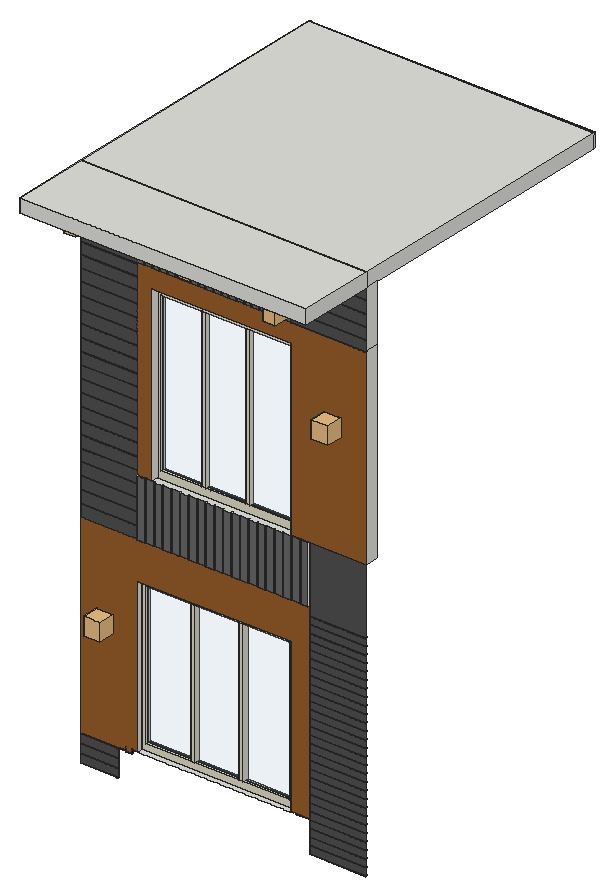
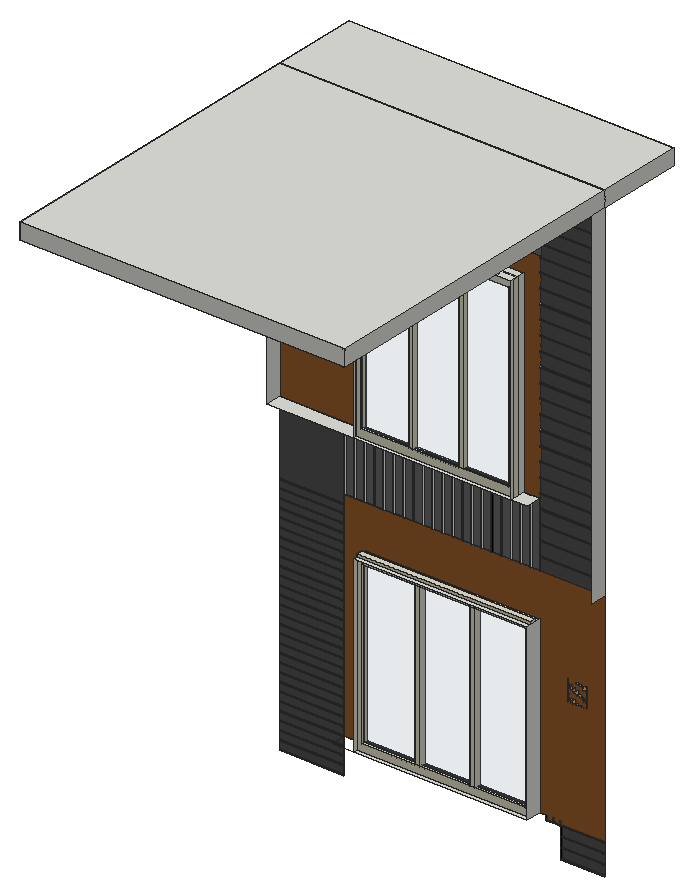
# SketchUp Ruby script. Lengths in inches.
U = 1.inch
M = Sketchup.active_model
def pt(a) = Geom::Point3d.new(a.map { |v| v * U })
def face(e, loops, mat)
  f = e.add_face(loops[0].map { |a| pt(a) })
  loops[1..].each { |l| e.add_face(l.map { |a| pt(a) }).erase! }
  f.material = f.back_material = mat if mat
  f
end
# faces: each face lists its corners as indices into pts; further lists are holes
def faces(e, pts, list, mat = nil) = list.each { |f| face(e, (f[0].is_a?(Array) ? f : [f]).map { |l| l.map { |i| pts[i] } }, mat) }
# xy, xz, yz: faces in a plane at the given z, y or x. An outline is a flat list of corners, or four numbers for a rectangle; further outlines are holes
def ring(l) = l.size == 4 ? [[l[0], l[1]], [l[2], l[1]], [l[2], l[3]], [l[0], l[3]]] : l.each_slice(2).to_a
def flat(e, list, mat, &to3) = list.each { |f| face(e, (f[0].is_a?(Array) ? f : [f]).map { |l| ring(l).map { |u, v| to3.(u, v) } }, mat) }
def xy(e, z, list, mat = nil) = flat(e, list, mat) { |x, y| [x, y, z] }
def xz(e, y, list, mat = nil) = flat(e, list, mat) { |x, z| [x, y, z] }
def yz(e, x, list, mat = nil) = flat(e, list, mat) { |y, z| [x, y, z] }
def lines(e, pts, list) = list.each { |a, b| e.add_line(pt(pts[a]), pt(pts[b])) }
# prism: a flat outline (further loops are holes) pulled along v
def prism(e, loops, v, mat = nil)
  f = face(e, loops, mat); d = Geom::Vector3d.new(v.map { |x| x * U })
  f.pushpull(f.normal.samedirection?(d) ? d.length : -d.length)
end
def box(e, o, s, mat = nil) = prism(e, [[o, [o[0] + s[0], o[1], o[2]], [o[0] + s[0], o[1] + s[1], o[2]], [o[0], o[1] + s[1], o[2]]]], [0, 0, s[2]], mat)
def at(x, y, z, deg = 0) = Geom::Transformation.translation(pt([x, y, z])) * Geom::Transformation.rotation(ORIGIN, Z_AXIS, deg.degrees)
def axes(o, x, y, z) = Geom::Transformation.new([*x, 0, *y, 0, *z, 0, *pt(o).to_a, 1])
def part(name) = M.definitions.add(name)
# library, detail: a bought-in or finely detailed component or shape, given as its bounding box
def library(name, o, s) = part(name).tap { |d| box(d.entities, o, s) }
def detail(e, o, s) = box(e.add_group.entities, o, s)
def put(e, d, t, mat = nil) = e.add_instance(d, t).tap { |i| i.material = mat if mat }
def group(e, t, mat = nil) = e.add_group.tap { |g| g.transformation = t; g.material = mat if mat }.entities
root = M.entities
M.materials.add("Glass").color = [171, 209, 242]
M.materials["Glass"].alpha = 0.09
M.materials.add("Plastic_SSS_01_White").color = [225, 221, 201]
M.materials.add("[0010_Snow]").color = [255, 250, 250]
M.materials.add("[0134_DimGray]").color = [105, 105, 105]
M.materials.add("[0135_DarkGray]").color = [81, 81, 81]
M.materials.add("[0137_Black]").color = [0, 0, 0]
M.materials.add("[Wood Floor Dark]1").color = [153, 94, 42]
c1 = part("Window frame")
xy(c1.entities,0,[[[104.47,83.98,176.47,131.98],[106.47,85.98,174.47,129.98]],[127.47,85.98,129.47,129.98],[150.47,85.98,152.47,129.98]],"Plastic_SSS_01_White")
xy(c1.entities,2,[[[104.47,83.98,176.47,131.98],[106.47,85.98,174.47,129.98]],[127.47,85.98,129.47,129.98],[150.47,85.98,152.47,129.98]],"Plastic_SSS_01_White")
xz(c1.entities,83.98,[[104.47,0,176.47,2]],"Plastic_SSS_01_White")
xz(c1.entities,85.98,[[106.47,0,127.47,2],[127.47,0,129.47,2],[129.47,0,150.47,2],[150.47,0,152.47,2],[152.47,0,174.47,2]],"Plastic_SSS_01_White")
xz(c1.entities,129.98,[[106.47,0,127.47,2],[127.47,0,129.47,2],[129.47,0,150.47,2],[150.47,0,152.47,2],[152.47,0,174.47,2]],"Plastic_SSS_01_White")
xz(c1.entities,131.98,[[104.47,0,176.47,2]],"Plastic_SSS_01_White")
yz(c1.entities,104.47,[[83.98,0,131.98,2]],"Plastic_SSS_01_White")
yz(c1.entities,106.47,[[85.98,0,129.98,2]],"Plastic_SSS_01_White")
yz(c1.entities,127.47,[[85.98,0,129.98,2]],"Plastic_SSS_01_White")
yz(c1.entities,129.47,[[85.98,0,129.98,2]],"Plastic_SSS_01_White")
yz(c1.entities,150.47,[[85.98,0,129.98,2]],"Plastic_SSS_01_White")
yz(c1.entities,152.47,[[85.98,0,129.98,2]],"Plastic_SSS_01_White")
yz(c1.entities,174.47,[[85.98,0,129.98,2]],"Plastic_SSS_01_White")
yz(c1.entities,176.47,[[83.98,0,131.98,2]],"Plastic_SSS_01_White")
c2 = part("Window pane")
box(c2.entities,[0,0,0],[67.88,44,0.5])
c3 = part("Glazed window assembly")
put(c3.entities,c1,at(-104.47,-83.98,0))
put(c3.entities,c2,at(2,2,0.7),"Glass")
c4 = part("window")
p = [[-596.28,88.12,20.39],[-668.28,88.12,20.39]]
lines(c4.entities,p,[[0,1]])
put(c4.entities,c3,axes([-668.28,88.12,20.39],[1,0,0],[0,0,1],[0,-1,0]))
c5 = library("Spot Light",[-5.1,-5.1,-11.05],[10.2,10.2,11.05])
c6 = library("Spot Light\#1",[-5.1,-5.1,-11.05],[10.2,10.2,11.05])
c7 = library("Sphere Light\#2",[-7.69,-7.69,-7.69],[15.38,15.38,15.38])
c8 = library("Sphere Light",[-0.01,-0.01,-0.01],[0.02,0.02,0.02])
c9 = library("Sphere Light\#1",[-0.01,-0.01,-0.01],[0.02,0.02,0.02])
xy(root,272.3,[[144.5,47.5,180,48]],"[0135_DarkGray]")
xy(root,272.8,[[144.5,47.5,180,48]],"[0135_DarkGray]")
xy(root,272.95,[[0,47.5,24,48]],"[0135_DarkGray]")
xy(root,273.45,[[0,47.5,24,48]],"[0135_DarkGray]")
xy(root,277.1,[[144.5,47.5,180,48]],"[0135_DarkGray]")
xy(root,277.6,[[144.5,47.5,180,48]],"[0135_DarkGray]")
xy(root,278.45,[[0,47.5,24,48]],"[0135_DarkGray]")
xy(root,278.95,[[0,47.5,24,48]],"[0135_DarkGray]")
xy(root,281.9,[[144.5,47.5,180,48]],"[0135_DarkGray]")
xy(root,282.4,[[144.5,47.5,180,48]],"[0135_DarkGray]")
xy(root,283.95,[[0,47.5,24,48]],"[0135_DarkGray]")
xy(root,284.45,[[0,47.5,24,48]],"[0135_DarkGray]")
xy(root,286.7,[[144.5,47.5,180,48]],"[0135_DarkGray]")
xy(root,287.2,[[144.5,47.5,180,48]],"[0135_DarkGray]")
xy(root,289.45,[[0,47.5,24,48]],"[0135_DarkGray]")
xy(root,291.5,[[144.5,47.5,180,48]],"[0135_DarkGray]")
xy(root,292,[[32.5,47.5,36,47.5,36,48,36.5,48,36.5,47.5,40,47.5,40,48,40.5,48,40.5,47.5,44,47.5,44,48,44.5,48,44.5,47.5,48,47.5,48,48,48.5,48,48.5,47.5,52,47.5,52,48,52.5,48,52.5,47.5,56,47.5,56,48,56.5,48,56.5,47.5,60,47.5,60,48,60.5,48,60.5,47.5,64,47.5,64,48,64.5,48,64.5,47.5,68,47.5,68,48,68.5,48,68.5,47.5,72,47.5,72,48,72.5,48,72.5,47.5,76,47.5,76,48,76.5,48,76.5,47.5,80,47.5,80,48,80.5,48,80.5,47.5,84,47.5,84,48,84.5,48,84.5,47.5,88,47.5,88,48,88.5,48,88.5,47.5,92,47.5,92,48,92.5,48,92.5,47.5,96,47.5,96,48,96.5,48,96.5,47.5,100,47.5,100,48,100.5,48,100.5,47.5,104,47.5,104,48,104.5,48,104.5,47.5,108,47.5,108,48,108.5,48,108.5,47.5,112,47.5,112,48,112.5,48,112.5,47.5,116,47.5,116,48,116.5,48,116.5,47.5,120,47.5,120,48,120.5,48,120.5,47.5,124,47.5,124,48,124.5,48,124.5,47.5,128,47.5,128,48,128.5,48,128.5,47.5,132,47.5,132,56.5,36,56.5,36,48,32.5,48],[132.5,47.5,136,48],[136.5,47.5,140,48],[140.5,47.5,144,48]])
xy(root,292,[[144.5,47.5,180,48]],"[0135_DarkGray]")
xy(root,296.3,[[144.5,47.5,180,48]],"[0135_DarkGray]")
xy(root,296.8,[[144.5,47.5,180,48]],"[0135_DarkGray]")
xy(root,301.1,[[144.5,47.5,180,48]],"[0135_DarkGray]")
xy(root,301.6,[[144.5,47.5,180,48]],"[0135_DarkGray]")
xy(root,305.9,[[144.5,47.5,180,48]],"[0135_DarkGray]")
xy(root,306.4,[[144.5,47.5,180,48]],"[0135_DarkGray]")
xy(root,310.7,[[144.5,47.5,180,48]],"[0135_DarkGray]")
xy(root,311.2,[[144.5,47.5,180,48]],"[0135_DarkGray]")
xy(root,315.5,[[144.5,47.5,180,48]],"[0135_DarkGray]")
xy(root,316,[[144.5,47.5,180,48]],"[0135_DarkGray]")
xy(root,320.3,[[144.5,47.5,180,48]],"[0135_DarkGray]")
xy(root,320.8,[[144.5,47.5,180,48]],"[0135_DarkGray]")
xy(root,325.1,[[144.5,47.5,180,48]],"[0135_DarkGray]")
xy(root,325.6,[[144.5,47.5,180,48]],"[0135_DarkGray]")
xy(root,329.9,[[144.5,47.5,180,48]],"[0135_DarkGray]")
xy(root,330.4,[[144.5,47.5,180,48]],"[0135_DarkGray]")
xy(root,334.7,[[144.5,47.5,180,48]],"[0135_DarkGray]")
xy(root,335.2,[[144.5,47.5,180,48]],"[0135_DarkGray]")
xy(root,339.5,[[144.5,47.5,180,48]],"[0135_DarkGray]")
xy(root,340,[[144.5,47.5,180,48]],"[0135_DarkGray]")
xy(root,344.3,[[144.5,47.5,180,48]],"[0135_DarkGray]")
xy(root,344.8,[[144.5,47.5,180,48]],"[0135_DarkGray]")
xy(root,349.1,[[144.5,47.5,180,48]],"[0135_DarkGray]")
xy(root,349.6,[[144.5,47.5,180,48]],"[0135_DarkGray]")
xy(root,353.9,[[144.5,47.5,180,48]],"[0135_DarkGray]")
xy(root,354.4,[[144.5,47.5,180,48]],"[0135_DarkGray]")
xy(root,358.7,[[144.5,47.5,180,48]],"[0135_DarkGray]")
xy(root,359.2,[[144.5,47.5,180,48]],"[0135_DarkGray]")
xy(root,363.5,[[144.5,47.5,180,48]],"[0135_DarkGray]")
xy(root,364,[[144.5,47.5,180,48]],"[0135_DarkGray]")
xy(root,368.3,[[144.5,47.5,180,48]],"[0135_DarkGray]")
xy(root,368.8,[[144.5,47.5,180,48]],"[0135_DarkGray]")
xy(root,373.1,[[144.5,47.5,180,48]],"[0135_DarkGray]")
xy(root,373.6,[[144.5,47.5,180,48]],"[0135_DarkGray]")
xy(root,377.9,[[144.5,47.5,180,48]],"[0135_DarkGray]")
xy(root,378.4,[[144.5,47.5,180,48]],"[0135_DarkGray]")
xy(root,382.7,[[144.5,47.5,180,48]],"[0135_DarkGray]")
xy(root,383.2,[[144.5,47.5,180,48]],"[0135_DarkGray]")
xy(root,387.5,[[144.5,47.5,180,48]],"[0135_DarkGray]")
xy(root,388,[[36,48,132,56.5]])
xy(root,388,[[144.5,47.5,180,48]],"[0135_DarkGray]")
xy(root,392.3,[[144.5,47.5,180,48]],"[0135_DarkGray]")
xy(root,392.8,[[144.5,47.5,180,48]],"[0135_DarkGray]")
xy(root,397.1,[[144.5,47.5,180,48]],"[0135_DarkGray]")
xy(root,397.6,[[144.5,47.5,180,48]],"[0135_DarkGray]")
xy(root,401.9,[[144.5,47.5,180,48]],"[0135_DarkGray]")
xy(root,402.4,[[144.5,47.5,180,48]],"[0135_DarkGray]")
xy(root,406.7,[[144.5,47.5,180,48]],"[0135_DarkGray]")
xy(root,407.2,[[144.5,47.5,180,48]],"[0135_DarkGray]")
xy(root,412,[[35.8125,47.5,40.73,48],[41.23,47.5,46.15,48],[46.65,47.5,51.57,48],[52.07,47.5,56.99,48],[57.49,47.5,62.41,48],
  [62.91,47.5,67.82,48],[68.32,47.5,73.24,48],[73.74,47.5,78.66,48],[79.16,47.5,84.08,48],[84.58,47.5,89.5,48],
  [90,47.5,94.92,48],[95.42,47.5,100.34,48],[100.84,47.5,105.76,48],[106.26,47.5,111.18,48],[111.68,47.5,116.59,48],
  [117.09,47.5,122.01,48],[122.51,47.5,127.43,48],[127.93,47.5,132.85,48],[133.35,47.5,138.27,48],[138.77,47.5,143.6875,48]],"[0010_Snow]")
xy(root,419.32,[[0,48,35.3125,48.5]],"[0010_Snow]")
xy(root,419.82,[[0,48,35.3125,48.5]],"[0010_Snow]")
xy(root,427.15,[[0,48,35.3125,48.5]],"[0010_Snow]")
xy(root,427.65,[[0,48,35.3125,48.5]],"[0010_Snow]")
xy(root,434.98,[[0,48,35.3125,48.5]],"[0010_Snow]")
xy(root,435.48,[[0,48,35.3125,48.5]],"[0010_Snow]")
xy(root,442.8,[[0,48,35.3125,48.5]],"[0010_Snow]")
xy(root,443.3,[[0,48,35.3125,48.5]],"[0010_Snow]")
xy(root,448,[[35.8125,47.5,40.73,48],[41.23,47.5,46.15,47.5,46.15,48,46.65,48,46.65,47.5,51.57,47.5,51.57,48,52.07,48,52.07,47.5,56.99,47.5,56.99,48,57.49,48,57.49,47.5,62.41,47.5,62.41,48,62.91,48,62.91,47.5,67.82,47.5,67.82,48,68.32,48,68.32,47.5,73.24,47.5,73.24,48,73.74,48,73.74,47.5,78.66,47.5,78.66,48,79.16,48,79.16,47.5,84.08,47.5,84.08,48,84.58,48,84.58,47.5,89.5,47.5,89.5,48,90,48,90,47.5,94.92,47.5,94.92,48,95.42,48,95.42,47.5,100.34,47.5,100.34,48,100.84,48,100.84,47.5,105.76,47.5,105.76,48,106.26,48,106.26,47.5,111.18,47.5,111.18,48,111.68,48,111.68,47.5,116.59,47.5,116.59,48,117.09,48,117.09,47.5,122.01,47.5,122.01,48,122.51,48,122.51,47.5,127.43,47.5,127.43,48,127.93,48,127.93,47.5,132.85,47.5,132.85,48,132,48,132,56.5,44.8,56.5,44.8,48,41.23,48],[133.35,47.5,138.27,48],[138.77,47.5,143.6875,48],[144.5,47.5,180,48],
  [35.8125,48,44.8,56.5],[132,48,180,56.5]])
xy(root,450.625,[[0,48,35.3125,48.5]],"[0010_Snow]")
xy(root,451.125,[[0,48,35.3125,48.5]],"[0010_Snow]")
xy(root,458.45,[[0,48,35.3125,48.5]],"[0010_Snow]")
xy(root,458.95,[[0,48,35.3125,48.5]],"[0010_Snow]")
xy(root,466.28,[[0,48,35.3125,48.5]],"[0010_Snow]")
xy(root,466.78,[[0,48,35.3125,48.5]],"[0010_Snow]")
xy(root,474.1,[[0,48,35.3125,48.5]],"[0010_Snow]")
xy(root,474.6,[[0,48,35.3125,48.5]],"[0010_Snow]")
xy(root,481.92,[[0,48,35.3125,48.5]],"[0010_Snow]")
xy(root,482.42,[[0,48,35.3125,48.5]],"[0010_Snow]")
xy(root,489.75,[[0,48,35.3125,48.5]],"[0010_Snow]")
xy(root,490.25,[[0,48,35.3125,48.5]],"[0010_Snow]")
xy(root,497.58,[[0,48,35.3125,48.5]],"[0010_Snow]")
xy(root,498.08,[[0,48,35.3125,48.5]],"[0010_Snow]")
xy(root,505.4,[[0,48,35.3125,48.5]],"[0010_Snow]")
xy(root,505.9,[[0,48,35.3125,48.5]],"[0010_Snow]")
xy(root,513.22,[[0,48,35.3125,48.5]],"[0010_Snow]")
xy(root,513.72,[[0,48,35.3125,48.5]],"[0010_Snow]")
xy(root,521.05,[[0,48,35.3125,48.5]],"[0010_Snow]")
xy(root,521.55,[[0,48,35.3125,48.5]],"[0010_Snow]")
xy(root,528.875,[[0,48,35.3125,48.25]],"[0010_Snow]")
xy(root,529.375,[[0,48,35.3125,48.25]],"[0010_Snow]")
xy(root,536.7,[[0,48,35.3125,48.25]],"[0010_Snow]")
xy(root,537.2,[[0,48,35.3125,48.25]],"[0010_Snow]")
xy(root,544.55,[[0,48,35.3125,48.5]],"[0010_Snow]")
xy(root,545.03,[[0,48,35.3125,48.5]],"[0010_Snow]")
xy(root,552.35,[[0,48,35.3125,48.5]],"[0010_Snow]")
xy(root,552.85,[[0,48,35.3125,48.5]],"[0010_Snow]")
xy(root,556.5,[[44.8,48,132,56.5]])
xy(root,560.17,[[0,48,35.3125,48.5]],"[0010_Snow]")
xy(root,560.67,[[0,48,35.3125,48.5]],"[0010_Snow]")
xy(root,567.5,[[0,48,35.3125,48.5]],"[0010_Snow]")
xy(root,568,[[0,48,35.3125,48.5],[132,48,180,48.5]],"[0010_Snow]")
xy(root,568.5,[[39.65,48,40.15,48.5],[44.48,48,44.98,48.5],[49.32,48,49.82,48.5],[54.15,48,54.65,48.5],[58.98,48,59.48,48.5],
  [63.82,48,64.32,48.5],[68.65,48,69.15,48.5],[73.49,48,73.99,48.5],[78.32,48,78.82,48.5],[83.16,48,83.66,48.5],
  [87.99,48,88.49,48.5],[92.83,48,93.33,48.5],[97.66,48,98.16,48.5],[102.49,48,102.99,48.5],[107.33,48,107.83,48.5],
  [112.16,48,112.66,48.5],[117,48,117.5,48.5],[121.83,48,122.33,48.5],[126.67,48,127.17,48.5],[132,48,180,48.5]],"[0010_Snow]")
xy(root,574.5,[[0,48,35.3125,48.5],[132,48,180,48.5]],"[0010_Snow]")
xy(root,575,[[0,48,35.3125,48.5],[132,48,180,48.5]],"[0010_Snow]")
xy(root,582,[[0,48,35.3125,48.5],[132,48,180,48.5]],"[0010_Snow]")
xy(root,582.5,[[0,48,35.3125,48.5],[132,48,180,48.5]],"[0010_Snow]")
xy(root,589.5,[[0,48,35.3125,48.5],[132,48,180,48.5]],"[0010_Snow]")
xy(root,590,[[0,48,35.3125,48.5],[132,48,180,48.5]],"[0010_Snow]")
xy(root,597,[[0,48,35.3125,48.5],[132,48,180,48.5]],"[0010_Snow]")
xy(root,597.5,[[0,48,35.3125,48.5],[132,48,180,48.5]],"[0010_Snow]")
xy(root,604.5,[[0,0,180,48],[0,48,0,56.5,180,56.5,180,48,127.17,48,127.17,48.5,126.67,48.5,126.67,48,122.33,48,122.33,48.5,121.83,48.5,121.83,48,117.5,48,117.5,48.5,117,48.5,117,48,112.66,48,112.66,48.5,112.16,48.5,112.16,48,107.83,48,107.83,48.5,107.33,48.5,107.33,48,102.99,48,102.99,48.5,102.49,48.5,102.49,48,98.16,48,98.16,48.5,97.66,48.5,97.66,48,93.33,48,93.33,48.5,92.83,48.5,92.83,48,88.49,48,88.49,48.5,87.99,48.5,87.99,48,83.66,48,83.66,48.5,83.16,48.5,83.16,48,78.82,48,78.82,48.5,78.32,48.5,78.32,48,73.99,48,73.99,48.5,73.49,48.5,73.49,48,69.15,48,69.15,48.5,68.65,48.5,68.65,48,64.32,48,64.32,48.5,63.82,48.5,63.82,48,59.48,48,59.48,48.5,58.98,48.5,58.98,48,54.65,48,54.65,48.5,54.15,48.5,54.15,48,49.82,48,49.82,48.5,49.32,48.5,49.32,48,44.98,48,44.98,48.5,44.48,48.5,44.48,48,40.15,48,40.15,48.5,39.65,48.5,39.65,48],[39.65,48,40.15,48.5],[44.48,48,44.98,48.5],[49.32,48,49.82,48.5],
  [54.15,48,54.65,48.5],[58.98,48,59.48,48.5],[63.82,48,64.32,48.5],[68.65,48,69.15,48.5],[73.49,48,73.99,48.5],
  [78.32,48,78.82,48.5],[83.16,48,83.66,48.5],[87.99,48,88.49,48.5],[92.83,48,93.33,48.5],[97.66,48,98.16,48.5],
  [102.49,48,102.99,48.5],[107.33,48,107.83,48.5],[112.16,48,112.66,48.5],[117,48,117.5,48.5],[121.83,48,122.33,48.5],
  [126.67,48,127.17,48.5],[0,56.5,0,227.5,180,227.5,180,56.5,171,56.5,171,218.5,9,218.5,9,56.5],[9,56.5,171,218.5],[0,227.5,180,227.75]])
xy(root,613.5,[[0,0,180,48],[0,48,180,227.5],[0,227.5,180,227.75]])
xz(root,0,[[0,604.5,180,613.5]])
xz(root,47.5,[[35.8125,412,40.73,448],[41.23,412,46.15,448],[46.65,412,51.57,448],[52.07,412,56.99,448],[57.49,412,62.41,448],
  [62.91,412,67.82,448],[68.32,412,73.24,448],[73.74,412,78.66,448],[79.16,412,84.08,448],[84.58,412,89.5,448],
  [90,412,94.92,448],[95.42,412,100.34,448],[100.84,412,105.76,448],[106.26,412,111.18,448],[111.68,412,116.59,448],
  [117.09,412,122.01,448],[122.51,412,127.43,448],[127.93,412,132.85,448],[133.35,412,138.27,448],[138.77,412,143.6875,448]],"[0134_DimGray]")
xz(root,47.5,[[144.5,272.8,180,277.1],[0,273.45,24,278.45],[144.5,277.6,180,281.9],[0,278.95,24,283.95],[144.5,282.4,180,286.7],
  [0,284.45,24,289.45],[144.5,287.2,180,291.5],[144.5,292,180,296.3],[144.5,296.8,180,301.1],[144.5,301.6,180,305.9],
  [144.5,306.4,180,310.7],[144.5,311.2,180,315.5],[144.5,316,180,320.3],[144.5,320.8,180,325.1],[144.5,325.6,180,329.9],
  [144.5,330.4,180,334.7],[144.5,335.2,180,339.5],[144.5,340,180,344.3],[144.5,344.8,180,349.1],[144.5,349.6,180,353.9],
  [144.5,354.4,180,358.7],[144.5,359.2,180,363.5],[144.5,364,180,368.3],[144.5,368.8,180,373.1],[144.5,373.6,180,377.9],
  [144.5,378.4,180,382.7],[144.5,383.2,180,387.5],[144.5,388,180,392.3],[144.5,392.8,180,397.1],[144.5,397.6,180,401.9],
  [144.5,402.4,180,406.7],[144.5,407.2,180,448]],"[0135_DarkGray]")
xz(root,48,[[0,604.5,180,613.5]])
xz(root,48,[[35.3125,568.5,39.65,604.5],[40.15,568.5,44.48,604.5],[44.98,568.5,49.32,604.5],[49.82,568.5,54.15,604.5],[54.65,568.5,58.98,604.5],
  [59.48,568.5,63.82,604.5],[64.32,568.5,68.65,604.5],[69.15,568.5,73.49,604.5],[73.99,568.5,78.32,604.5],[78.82,568.5,83.16,604.5],
  [83.66,568.5,87.99,604.5],[88.49,568.5,92.83,604.5],[93.33,568.5,97.66,604.5],[98.16,568.5,102.49,604.5],[102.99,568.5,107.33,604.5],
  [107.83,568.5,112.16,604.5],[112.66,568.5,117,604.5],[117.5,568.5,121.83,604.5],[122.33,568.5,126.67,604.5],[127.17,568.5,132,604.5]],"[0134_DimGray]")
xz(root,48,[[144.5,272.3,180,272.8],[0,272.95,24,273.45],[144.5,277.1,180,277.6],[0,278.45,24,278.95],[144.5,281.9,180,282.4],
  [0,283.95,24,284.45],[144.5,286.7,180,287.2],[0,289.45,24,289.95],[144.5,291.5,180,292],[144.5,296.3,180,296.8],
  [144.5,301.1,180,301.6],[144.5,305.9,180,306.4],[144.5,310.7,180,311.2],[144.5,315.5,180,316],[144.5,320.3,180,320.8],
  [144.5,325.1,180,325.6],[144.5,329.9,180,330.4],[144.5,334.7,180,335.2],[144.5,339.5,180,340],[144.5,344.3,180,344.8],
  [144.5,349.1,180,349.6],[144.5,353.9,180,354.4],[144.5,358.7,180,359.2],[144.5,363.5,180,364],[144.5,368.3,180,368.8],
  [144.5,373.1,180,373.6],[144.5,377.9,180,378.4],[144.5,382.7,180,383.2],[144.5,387.5,180,388],[144.5,392.3,180,392.8],
  [144.5,397.1,180,397.6],[144.5,401.9,180,402.4],[144.5,406.7,180,407.2],[0,412,35.3125,419.32],[0,419.82,35.3125,427.15],
  [0,427.65,35.3125,434.98],[0,435.48,35.3125,442.8],[0,443.3,35.3125,450.625],[0,451.125,35.3125,458.45],[0,458.95,35.3125,466.28],
  [0,466.78,35.3125,474.1],[0,474.6,35.3125,481.92],[0,482.42,35.3125,489.75],[0,490.25,35.3125,497.58],[0,498.08,35.3125,505.4],
  [0,505.9,35.3125,513.22],[0,513.72,35.3125,521.05],[0,521.55,35.3125,528.875],[0,529.375,35.3125,536.7],[0,537.2,35.3125,544.55],
  [0,545.03,35.3125,552.35],[0,552.85,35.3125,560.17],[0,560.67,35.3125,567.5],[0,568,35.3125,574.5],[132,568.5,180,574.5],
  [0,575,35.3125,582],[132,575,180,582],[0,582.5,35.3125,589.5],[132,582.5,180,589.5],[0,590,35.3125,597],
  [132,590,180,597],[0,597.5,35.3125,604.5],[132,597.5,180,604.5]],"[0135_DarkGray]")
xz(root,48,[[32,289.45,32.5,289.95],[32,289.95,32.5,292],[40.73,412,41.23,448],[46.15,412,46.65,448],[51.57,412,52.07,448],
  [56.99,412,57.49,448],[62.41,412,62.91,448],[67.82,412,68.32,448],[73.24,412,73.74,448],[78.66,412,79.16,448],
  [84.08,412,84.58,448],[89.5,412,90,448],[94.92,412,95.42,448],[100.34,412,100.84,448],[105.76,412,106.26,448],
  [111.18,412,111.68,448],[116.59,412,117.09,448],[122.01,412,122.51,448],[127.43,412,127.93,448],[132.85,412,133.35,448],
  [138.27,412,138.77,448]],"[0137_Black]")
xz(root,48,[[24,289.45,24.5,289.95],[24.5,289.45,28,289.95],[28,289.45,28.5,289.95],[28.5,289.45,32,289.95],[0,289.95,24,289.95,24,292,24.5,292,24.5,289.95,28,289.95,28,292,28.5,292,28.5,289.95,32,289.95,32,292,36,292,36,388,132,388,132,292,144,292,143.6875,412,0,412],
  [24,289.95,24.5,292],[28,289.95,28.5,292],[35.3125,412,35.8125,412,35.8125,448,44.8,448,44.8,556.5,132,556.5,132,448,180,448,180,568,132,568,132,568.5,35.3125,568.5]],"[Wood Floor Dark]1")
xz(root,48.25,[[0,528.875,35.3125,529.375],[0,536.7,35.3125,537.2]],"[0010_Snow]")
xz(root,48.5,[[0,458.45,35.3125,458.95],[0,466.28,35.3125,466.78],[0,474.1,35.3125,474.6],[0,481.92,35.3125,482.42],[0,489.75,35.3125,490.25],
  [0,497.58,35.3125,498.08],[0,505.4,35.3125,505.9],[0,513.22,35.3125,513.72],[0,521.05,35.3125,521.55],[0,544.55,35.3125,545.03],
  [0,552.35,35.3125,552.85],[0,560.17,35.3125,560.67],[0,567.5,35.3125,568],[0,574.5,35.3125,575],[0,582,35.3125,582.5]],"[0010_Snow]")
xz(root,48.5,[[0,419.32,35.3125,419.82],[0,427.15,35.3125,427.65],[0,434.98,35.3125,435.48],[0,442.8,35.3125,443.3],[0,450.625,35.3125,451.125],
  [132,568,180,568.5],[39.65,568.5,40.15,604.5],[44.48,568.5,44.98,604.5],[49.32,568.5,49.82,604.5],[54.15,568.5,54.65,604.5],
  [58.98,568.5,59.48,604.5],[63.82,568.5,64.32,604.5],[68.65,568.5,69.15,604.5],[73.49,568.5,73.99,604.5],[78.32,568.5,78.82,604.5],
  [83.16,568.5,83.66,604.5],[87.99,568.5,88.49,604.5],[92.83,568.5,93.33,604.5],[97.66,568.5,98.16,604.5],[102.49,568.5,102.99,604.5],
  [107.33,568.5,107.83,604.5],[112.16,568.5,112.66,604.5],[117,568.5,117.5,604.5],[121.83,568.5,122.33,604.5],[126.67,568.5,127.17,604.5],
  [132,574.5,180,575],[132,582,180,582.5],[0,589.5,35.3125,590],[132,589.5,180,590],[0,597,35.3125,597.5],
  [132,597,180,597.5]],"[0137_Black]")
xz(root,227.75,[[0,604.5,180,613.5]])
yz(root,0,[[48,412,48,419.32,48.5,419.32,48.5,419.82,48,419.82,48,427.15,48.5,427.15,48.5,427.65,48,427.65,48,434.98,48.5,434.98,48.5,435.48,48,435.48,48,442.8,48.5,442.8,48.5,443.3,48,443.3,48,450.625,48.5,450.625,48.5,451.125,48,451.125,48,458.45,48.5,458.45,48.5,458.95,48,458.95,48,466.28,48.5,466.28,48.5,466.78,48,466.78,48,474.1,48.5,474.1,48.5,474.6,48,474.6,48,481.92,48.5,481.92,48.5,482.42,48,482.42,48,489.75,48.5,489.75,48.5,490.25,48,490.25,48,497.58,48.5,497.58,48.5,498.08,48,498.08,48,505.4,48.5,505.4,48.5,505.9,48,505.9,48,513.22,48.5,513.22,48.5,513.72,48,513.72,48,521.05,48.5,521.05,48.5,521.55,48,521.55,48,528.875,48.25,528.875,48.25,529.375,48,529.375,48,536.7,48.25,536.7,48.25,537.2,48,537.2,48,544.55,48.5,544.55,48.5,545.03,48,545.03,48,552.35,48.5,552.35,48.5,552.85,48,552.85,48,560.17,48.5,560.17,48.5,560.67,48,560.67,48,567.5,48.5,567.5,48.5,568,48,568,48,574.5,48.5,574.5,48.5,575,48,575,48,582,48.5,582,48.5,582.5,48,582.5,48,589.5,48.5,589.5,48.5,590,48,590,48,597,48.5,597,48.5,597.5,48,597.5,48,604.5,56.5,604.5,56.5,412],[0,604.5,48,613.5],[48,604.5,227.5,613.5],[227.5,604.5,227.75,613.5]])
yz(root,24,[[47.5,273.45,48,278.45],[47.5,278.95,48,283.95],[47.5,284.45,48,289.45]],"[0137_Black]")
yz(root,35.3125,[[48,419.32,48.5,419.82],[48,427.15,48.5,427.65],[48,434.98,48.5,435.48],[48,442.8,48.5,443.3],[48,450.625,48.5,451.125],
  [48,458.45,48.5,458.95],[48,466.28,48.5,466.78],[48,474.1,48.5,474.6],[48,481.92,48.5,482.42],[48,489.75,48.5,490.25],
  [48,497.58,48.5,498.08],[48,505.4,48.5,505.9],[48,513.22,48.5,513.72],[48,521.05,48.5,521.55],[48,528.875,48.25,529.375],
  [48,536.7,48.25,537.2],[48,544.55,48.5,545.03],[48,552.35,48.5,552.85],[48,560.17,48.5,560.67],[48,567.5,48.5,568],
  [48,574.5,48.5,575],[48,582,48.5,582.5],[48,589.5,48.5,590],[48,597,48.5,597.5]],"[0010_Snow]")
yz(root,35.8125,[[47.5,412,48,448]],"[0010_Snow]")
yz(root,36,[[48,292,56.5,388]])
yz(root,39.65,[[48,568.5,48.5,604.5]],"[0010_Snow]")
yz(root,40.15,[[48,568.5,48.5,574.5],[48,574.5,48.5,604.5]],"[0010_Snow]")
yz(root,40.73,[[47.5,412,48,448]],"[0010_Snow]")
yz(root,41.23,[[47.5,412,48,448]],"[0010_Snow]")
yz(root,44.48,[[48,568.5,48.5,604.5]],"[0010_Snow]")
yz(root,44.8,[[48,448,56.5,556.5]])
yz(root,44.98,[[48,568.5,48.5,574.5],[48,574.5,48.5,604.5]],"[0010_Snow]")
yz(root,46.15,[[47.5,412,48,448]],"[0010_Snow]")
yz(root,46.65,[[47.5,412,48,448]],"[0010_Snow]")
yz(root,49.32,[[48,568.5,48.5,604.5]],"[0010_Snow]")
yz(root,49.82,[[48,568.5,48.5,574.5],[48,574.5,48.5,604.5]],"[0010_Snow]")
yz(root,51.57,[[47.5,412,48,448]],"[0010_Snow]")
yz(root,52.07,[[47.5,412,48,448]],"[0010_Snow]")
yz(root,54.15,[[48,568.5,48.5,604.5]],"[0010_Snow]")
yz(root,54.65,[[48,568.5,48.5,574.5],[48,574.5,48.5,604.5]],"[0010_Snow]")
yz(root,56.99,[[47.5,412,48,448]],"[0010_Snow]")
yz(root,57.49,[[47.5,412,48,448]],"[0010_Snow]")
yz(root,58.98,[[48,568.5,48.5,604.5]],"[0010_Snow]")
yz(root,59.48,[[48,568.5,48.5,574.5],[48,574.5,48.5,604.5]],"[0010_Snow]")
yz(root,62.41,[[47.5,412,48,448]],"[0137_Black]")
yz(root,62.91,[[47.5,412,48,448]],"[0010_Snow]")
yz(root,63.82,[[48,568.5,48.5,604.5]],"[0010_Snow]")
yz(root,64.32,[[48,568.5,48.5,574.5],[48,574.5,48.5,604.5]],"[0010_Snow]")
yz(root,67.82,[[47.5,412,48,448]],"[0010_Snow]")
yz(root,68.32,[[47.5,412,48,448]],"[0010_Snow]")
yz(root,68.65,[[48,568.5,48.5,604.5]],"[0010_Snow]")
yz(root,69.15,[[48,568.5,48.5,574.5],[48,574.5,48.5,604.5]],"[0010_Snow]")
yz(root,73.24,[[47.5,412,48,448]],"[0010_Snow]")
yz(root,73.49,[[48,568.5,48.5,604.5]],"[0010_Snow]")
yz(root,73.74,[[47.5,412,48,448]],"[0010_Snow]")
yz(root,73.99,[[48,568.5,48.5,574.5],[48,574.5,48.5,604.5]],"[0010_Snow]")
yz(root,78.32,[[48,568.5,48.5,604.5]],"[0010_Snow]")
yz(root,78.66,[[47.5,412,48,448]],"[0010_Snow]")
yz(root,78.82,[[48,568.5,48.5,574.5],[48,574.5,48.5,604.5]],"[0010_Snow]")
yz(root,79.16,[[47.5,412,48,448]],"[0010_Snow]")
yz(root,83.16,[[48,568.5,48.5,604.5]],"[0010_Snow]")
yz(root,83.66,[[48,568.5,48.5,574.5],[48,574.5,48.5,604.5]],"[0010_Snow]")
yz(root,84.08,[[47.5,412,48,448]],"[0010_Snow]")
yz(root,84.58,[[47.5,412,48,448]],"[0010_Snow]")
yz(root,87.99,[[48,568.5,48.5,604.5]],"[0010_Snow]")
yz(root,88.49,[[48,568.5,48.5,574.5],[48,574.5,48.5,604.5]],"[0010_Snow]")
yz(root,89.5,[[47.5,412,48,448]],"[0010_Snow]")
yz(root,90,[[47.5,412,48,448]],"[0010_Snow]")
yz(root,92.83,[[48,568.5,48.5,604.5]],"[0010_Snow]")
yz(root,93.33,[[48,568.5,48.5,574.5],[48,574.5,48.5,604.5]],"[0010_Snow]")
yz(root,94.92,[[47.5,412,48,448]],"[0010_Snow]")
yz(root,95.42,[[47.5,412,48,448]],"[0010_Snow]")
yz(root,97.66,[[48,568.5,48.5,604.5]],"[0010_Snow]")
yz(root,98.16,[[48,568.5,48.5,574.5],[48,574.5,48.5,604.5]],"[0010_Snow]")
yz(root,100.34,[[47.5,412,48,448]],"[0010_Snow]")
yz(root,100.84,[[47.5,412,48,448]],"[0010_Snow]")
yz(root,102.49,[[48,568.5,48.5,604.5]],"[0010_Snow]")
yz(root,102.99,[[48,568.5,48.5,574.5],[48,574.5,48.5,604.5]],"[0010_Snow]")
yz(root,105.76,[[47.5,412,48,448]],"[0010_Snow]")
yz(root,106.26,[[47.5,412,48,448]],"[0010_Snow]")
yz(root,107.33,[[48,568.5,48.5,604.5]],"[0010_Snow]")
yz(root,107.83,[[48,568.5,48.5,574.5],[48,574.5,48.5,604.5]],"[0010_Snow]")
yz(root,111.18,[[47.5,412,48,448]],"[0010_Snow]")
yz(root,111.68,[[47.5,412,48,448]],"[0010_Snow]")
yz(root,112.16,[[48,568.5,48.5,604.5]],"[0010_Snow]")
yz(root,112.66,[[48,568.5,48.5,574.5],[48,574.5,48.5,604.5]],"[0010_Snow]")
yz(root,116.59,[[47.5,412,48,448]],"[0010_Snow]")
yz(root,117,[[48,568.5,48.5,604.5]],"[0010_Snow]")
yz(root,117.09,[[47.5,412,48,448]],"[0010_Snow]")
yz(root,117.5,[[48,568.5,48.5,574.5],[48,574.5,48.5,604.5]],"[0010_Snow]")
yz(root,121.83,[[48,568.5,48.5,604.5]],"[0010_Snow]")
yz(root,122.01,[[47.5,412,48,448]],"[0010_Snow]")
yz(root,122.33,[[48,568.5,48.5,574.5],[48,574.5,48.5,604.5]],"[0010_Snow]")
yz(root,122.51,[[47.5,412,48,448]],"[0010_Snow]")
yz(root,126.67,[[48,568.5,48.5,604.5]],"[0010_Snow]")
yz(root,127.17,[[48,568.5,48.5,574.5],[48,574.5,48.5,604.5]],"[0010_Snow]")
yz(root,127.43,[[47.5,412,48,448]],"[0010_Snow]")
yz(root,127.93,[[47.5,412,48,448]],"[0010_Snow]")
yz(root,132,[[48,292,56.5,388],[48,448,56.5,556.5]])
yz(root,132,[[48,568,48.5,568.5],[48,574.5,48.5,575],[48,582,48.5,582.5],[48,589.5,48.5,590],[48,597,48.5,597.5]],"[0010_Snow]")
yz(root,132.85,[[47.5,412,48,448]],"[0010_Snow]")
yz(root,133.35,[[47.5,412,48,448]],"[0010_Snow]")
yz(root,138.27,[[47.5,412,48,448]],"[0010_Snow]")
yz(root,138.77,[[47.5,412,48,448]],"[0010_Snow]")
yz(root,143.6875,[[47.5,412,48,448]],"[0010_Snow]")
yz(root,144.5,[[47.5,272.8,48,277.1],[47.5,277.6,48,281.9],[47.5,282.4,48,286.7],[47.5,287.2,48,291.5],[47.5,292,48,296.3],
  [47.5,296.8,48,301.1],[47.5,301.6,48,305.9],[47.5,306.4,48,310.7],[47.5,311.2,48,315.5],[47.5,316,48,320.3],
  [47.5,320.8,48,325.1],[47.5,325.6,48,329.9],[47.5,330.4,48,334.7],[47.5,335.2,48,339.5],[47.5,340,48,344.3],
  [47.5,344.8,48,349.1],[47.5,349.6,48,353.9],[47.5,354.4,48,358.7],[47.5,359.2,48,363.5],[47.5,364,48,368.3],
  [47.5,368.8,48,373.1],[47.5,373.6,48,377.9],[47.5,378.4,48,382.7],[47.5,383.2,48,387.5],[47.5,388,48,392.3],
  [47.5,392.8,48,397.1],[47.5,397.6,48,401.9],[47.5,402.4,48,406.7],[47.5,407.2,48,448]],"[0135_DarkGray]")
yz(root,180,[[48,448,56.5,448,56.5,568.5,48.5,568.5,48.5,568,48,568],[48,568.5,56.5,568.5,56.5,604.5,48,604.5,48,597.5,48.5,597.5,48.5,597,48,597,48,590,48.5,590,48.5,589.5,48,589.5,48,582.5,48.5,582.5,48.5,582,48,582,48,575,48.5,575,48.5,574.5,48,574.5],[0,604.5,48,613.5],[48,604.5,227.5,613.5],[227.5,604.5,227.75,613.5]])
p = [[144,56.5,292],[132,56.5,292],[144,48,292]]
lines(root,p,[[0,1],[2,0]])
put(root,c4,axes([927.05,-93.78,250.58],[1.33333,0,0],[0,1.68,0],[0,0,2.03125]))
put(root,c5,at(14.9,42.9,363.82))
put(root,c4,axes([854.19,-59.15,401.9],[1.21116,0,0],[0,1.2936,0],[0,0,2.26042]))
put(root,c6,at(158.47,42.9,525.32))
put(root,c7,axes([156.96,7.69,601.04],[0.5,0,0],[0,1,0],[0,0,0.45]))
put(root,c7,axes([96.55,15.74,601.04],[0.5,0,0],[0,1,0],[0,0,0.45]))
put(root,c7,axes([25.12,15.74,601.04],[0.5,0,0],[0,1,0],[0,0,0.45]))
put(root,c8,at(154.36,18.44,604.5))
put(root,c9,at(154.36,18.44,604.5))
